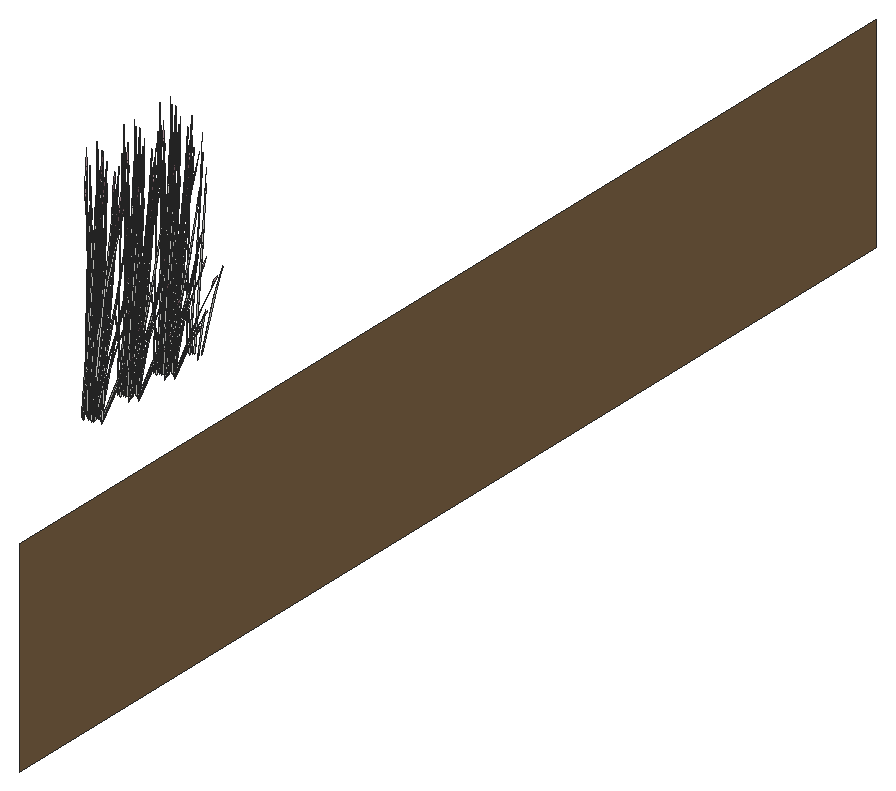
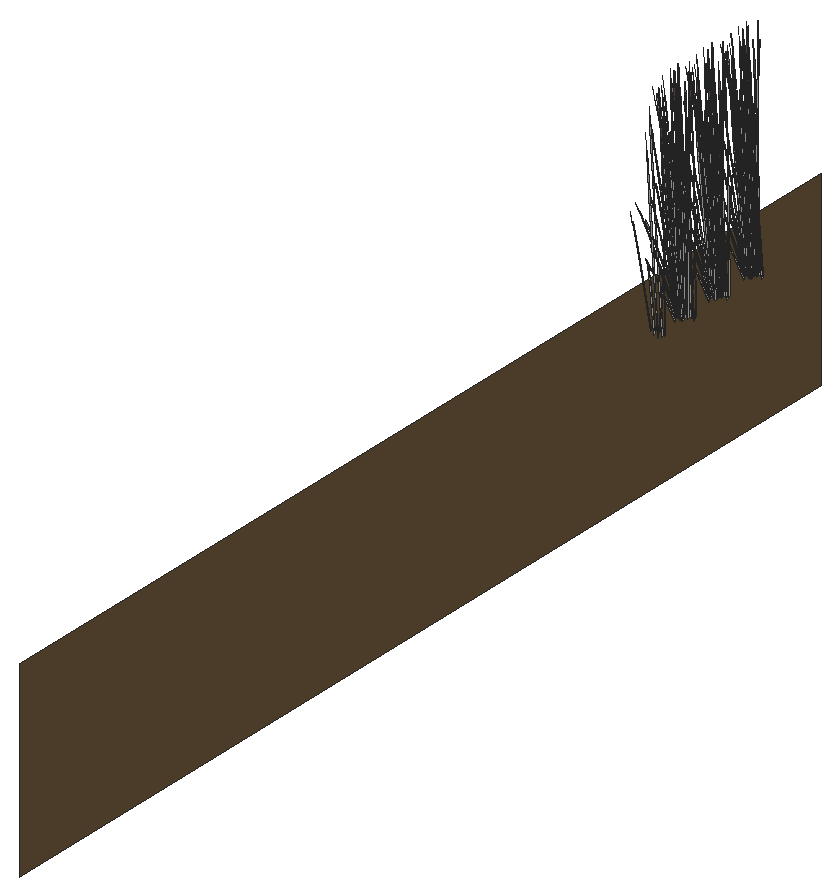
# SketchUp Ruby script. Lengths in inches.
U = 1.inch
M = Sketchup.active_model
def pt(a) = Geom::Point3d.new(a.map { |v| v * U })
def face(e, loops, mat)
  f = e.add_face(loops[0].map { |a| pt(a) })
  loops[1..].each { |l| e.add_face(l.map { |a| pt(a) }).erase! }
  f.material = f.back_material = mat if mat
  f
end
# faces: each face lists its corners as indices into pts; further lists are holes
def faces(e, pts, list, mat = nil) = list.each { |f| face(e, (f[0].is_a?(Array) ? f : [f]).map { |l| l.map { |i| pts[i] } }, mat) }
# xy, xz, yz: faces in a plane at the given z, y or x. An outline is a flat list of corners, or four numbers for a rectangle; further outlines are holes
def ring(l) = l.size == 4 ? [[l[0], l[1]], [l[2], l[1]], [l[2], l[3]], [l[0], l[3]]] : l.each_slice(2).to_a
def flat(e, list, mat, &to3) = list.each { |f| face(e, (f[0].is_a?(Array) ? f : [f]).map { |l| ring(l).map { |u, v| to3.(u, v) } }, mat) }
def xy(e, z, list, mat = nil) = flat(e, list, mat) { |x, y| [x, y, z] }
def xz(e, y, list, mat = nil) = flat(e, list, mat) { |x, z| [x, y, z] }
def yz(e, x, list, mat = nil) = flat(e, list, mat) { |y, z| [x, y, z] }
def lines(e, pts, list) = list.each { |a, b| e.add_line(pt(pts[a]), pt(pts[b])) }
# prism: a flat outline (further loops are holes) pulled along v
def prism(e, loops, v, mat = nil)
  f = face(e, loops, mat); d = Geom::Vector3d.new(v.map { |x| x * U })
  f.pushpull(f.normal.samedirection?(d) ? d.length : -d.length)
end
def box(e, o, s, mat = nil) = prism(e, [[o, [o[0] + s[0], o[1], o[2]], [o[0] + s[0], o[1] + s[1], o[2]], [o[0], o[1] + s[1], o[2]]]], [0, 0, s[2]], mat)
def at(x, y, z, deg = 0) = Geom::Transformation.translation(pt([x, y, z])) * Geom::Transformation.rotation(ORIGIN, Z_AXIS, deg.degrees)
def axes(o, x, y, z) = Geom::Transformation.new([*x, 0, *y, 0, *z, 0, *pt(o).to_a, 1])
def part(name) = M.definitions.add(name)
# library, detail: a bought-in or finely detailed component or shape, given as its bounding box
def library(name, o, s) = part(name).tap { |d| box(d.entities, o, s) }
def detail(e, o, s) = box(e.add_group.entities, o, s)
def put(e, d, t, mat = nil) = e.add_instance(d, t).tap { |i| i.material = mat if mat }
def group(e, t, mat = nil) = e.add_group.tap { |g| g.transformation = t; g.material = mat if mat }.entities
root = M.entities
M.materials.add("LightPink_Translucent").color = [144, 107, 117]
M.materials["LightPink_Translucent"].alpha = 0.75
M.materials.add("Soil_03_1K").color = [122, 96, 67]
c1 = part("blade")
p = [[2.15,0.21,22],[0,0.17,0],[0.09,0.45,0],[2.18,0.31,22],[2.29,0.31,22],[0.38,0.45,0],
  [2.48,0.24,33],[2.49,0.24,33],[2.48,0.22,33]]
faces(c1.entities,p,[[0,1,2,3],[4,5,2,3],[6,3,4,7],[8,0,3,6]])
c2 = part("seeds")
p = [[0.3,-0.1,1.38],[-0.01,-0.03,1.59],[-0.01,-0.03,0.03],[0.14,-0.07,-0.07],[0.29,-0.03,3],[0.15,0.01,3.11]]
faces(c2.entities,p,[[0,1,2,3],[1,0,4,5]],"LightPink_Translucent")
c3 = part("blade with seeds")
put(c3.entities,c1,at(0,0,0))
put(c3.entities,c2,axes([2.4,0.25,30.99],[1.5799,-0.05474,1.17369],[-0.12525,1.92788,0.29478],[-0.07173,-0.02425,1.56792]))
yz(root,352,[[262,0,514,48]],"Soil_03_1K")
put(root,c3,axes([333.35,303.47,49.78],[0.47255,-0.19538,-0.43871],[0.28245,0.35034,0],[0.10763,-0.0445,1.3917]))
put(root,c3,axes([336.15,304.15,50.29],[-0.18038,-0.01157,1.26356],[-0.18479,-0.31048,-0.27174],[0.22159,-0.08783,0.54024]))
put(root,c3,axes([333.91,304.28,49.82],[0.34009,-0.2937,-0.55095],[0.42248,0.26632,-0.1446],[0.13628,-0.07327,1.21613]))
put(root,c3,axes([333.54,304.62,50.36],[-0.05884,-0.44587,-0.25709],[0.6128,-0.02696,-0.44182],[0.10791,-0.05939,1.41118]))
put(root,c3,axes([333.46,303.63,49.79],[0.47106,0.09668,-0.27372],[-0.11861,0.34048,0.27372],[0.09497,-0.03926,1.22797]))
put(root,c3,axes([333.62,304.97,50.15],[0.56891,0.18939,0.21263],[-0.2738,0.39352,0.44182],[0,-0.09071,1.41855]))
put(root,c3,axes([333.44,304.7,50.4],[-0.54829,0.02412,0.39531],[-0.04958,-0.40041,-0.19025],[0.09816,-0.04058,1.26923]))
put(root,c3,axes([335.24,303.63,50.1],[0.31568,-0.39156,0],[0.52815,0.21836,-0.456],[0.12029,0.04973,1.44655]))
put(root,c3,axes([336.49,305.18,49.75],[-0.3252,0.04689,1.25103],[-0.05176,-0.37326,0.07161],[0.22777,-0.0565,0.71188]))
put(root,c3,axes([337.08,304.85,50],[-0.31304,-0.24986,-0.05733],[0.34284,-0.22894,-0.25992],[0.09714,-0.01612,0.85731]))
put(root,c3,axes([334.21,304.88,49.95],[0,-0.45213,0],[0.63136,0,0],[0,0,1.58567]))
put(root,c3,axes([334.97,303.84,50.19],[-0.47255,-0.19538,0.43871],[0.28245,-0.35034,0],[0.10763,0.0445,1.3917]))
put(root,c3,axes([333.91,304.6,50.09],[-0.41865,0.35461,0.40429],[-0.49737,-0.31303,0.15865],[0.10093,-0.03539,1.40366]))
put(root,c3,axes([333.18,304.01,50.1875],[-0.14586,0.38834,0.15589],[-0.53375,-0.1099,0.31002],[0.0922,-0.00189,1.41735]))
put(root,c3,axes([332.96,304.33,49.41],[-0.49699,0.15644,1.13921],[-0.15819,-0.44887,0.44265],[0.30518,0.00747,1.29573]))
put(root,c3,axes([334.29,304.45,50.3125],[0.09741,-0.34873,0.12794],[0.4759,0.06053,-0.36534],[0.08661,0.03581,1.11991]))
put(root,c3,axes([336.84,304.9375,49.32],[-0.02639,-0.05932,1.55816],[0.18302,-0.34702,-0.23804],[0.18462,-0.00499,0.26541]))
put(root,c3,axes([334.09,304.54,50.4],[-0.30332,-0.32798,0.39531],[0.45944,-0.23096,-0.19025],[0.09816,0.04058,1.26923]))
put(root,c3,axes([334.25,304.56,50.36],[0.50979,-0.25942,-0.25709],[0.339,0.36656,-0.44182],[0.12578,0.03723,1.41118]))
put(root,c3,axes([335.53,303.87,49.78],[0.47255,0.19538,-0.43871],[-0.28245,0.35034,0],[0.10763,0.0445,1.3917]))
put(root,c3,axes([334.63,304.98,49.95],[0.56491,0,0],[0,0.40454,0],[0,0,1.5764]))
put(root,c3,axes([334.79,304.04,50.1875],[-0.54257,0.10371,0.15589],[-0.13397,-0.38597,0.31002],[0.04839,0.05624,1.41735]))
put(root,c3,axes([335.4,304.02,49.79],[0.11861,0.34048,-0.27372],[-0.47106,0.09668,0.27372],[0.09497,0.03926,1.22797]))
put(root,c3,axes([334.45,304.78,50.1],[-0.63817,-0.08233,0.43472],[0.12987,-0.46497,0.17059],[0.09326,0.0449,1.50931]))
put(root,c3,axes([334.56,305.88,49.93],[0.53009,-0.13258,-0.16963],[0.18627,0.38191,0.00007],[0.05851,-0.01465,1.53656]))
put(root,c3,axes([334.62,305.16,49.96],[0.35245,0.2524,0],[-0.35245,0.2524,0],[0,0,1.49564]))
put(root,c3,axes([335.58,305.05,50.1875],[-0.39671,-0.28463,0.15589],[0.39978,-0.27607,0.31002],[-0.04381,0.05813,1.41735]))
put(root,c3,axes([334.84,304.62,49.82],[0.52523,0.06406,-0.55095],[-0.11084,0.39517,-0.1446],[0.15674,0.04788,1.21613]))
put(root,c3,axes([334.62,304.86,50.4],[0.24498,-0.3521,0.39531],[0.50902,0.16945,-0.19025],[0,0.08116,1.26923]))
put(root,c3,axes([334.52,305.0625,50.03],[0,0.45191,-0.04981],[-0.63136,0,0],[0,0.0142,1.58489]))
put(root,c3,axes([334.57,304.74,49.95],[0.30332,0.32798,-0.39531],[-0.45944,0.23096,0.19025],[0.09816,0.04058,1.26923]))
put(root,c3,axes([335.9,305.06,50.19],[0,-0.39075,0.43871],[0.56491,0,0],[0,0.089,1.3917]))
put(root,c3,axes([334.83,304.94,50.3125],[0.47043,-0.11396,0.12794],[0.16474,0.32541,-0.36534],[0,0.07162,1.11991]))
put(root,c3,axes([336.58,305.74,50.29],[-0.1216,-0.0961,1.26356],[0.15822,-0.31792,-0.27174],[0.24603,0.04307,0.54024]))
put(root,c3,axes([334.4,306.09,49.95],[0.50902,0.17543,0],[-0.24498,0.36452,0],[0,0,1.54589]))
put(root,c3,axes([334.22,305.9375,50.02],[0.21952,0.44891,-0.05313],[-0.62724,0.1573,0],[0.00767,0.01568,1.52132]))
put(root,c3,axes([336.29,305.125,50.1],[0.63136,0,0],[0,0.43672,-0.456],[0,0.09947,1.44655]))
put(root,c3,axes([336.03,305.35,49.94],[-0.63105,-0.00312,-0.04397],[0,-0.43672,0.44129],[-0.01983,0.09942,1.3992]))
put(root,c3,axes([334.67,304.97,50.36],[0.56863,0.18645,-0.25709],[-0.2738,0.39352,-0.44182],[0.01787,0.09662,1.41118]))
put(root,c3,axes([335.9,305.41,49.79],[-0.35245,0.2438,-0.27372],[-0.35245,-0.2438,0.27372],[0,0.07853,1.22797]))
put(root,c3,axes([336.15,305.42,49.78],[0,0.39075,-0.43871],[-0.56491,0,0],[0,0.089,1.3917]))
put(root,c3,axes([335.51,306.65,49.32],[0.03679,-0.05641,1.55816],[0.46313,-0.16615,-0.23804],[0.14041,0.08599,0.26541]))
put(root,c3,axes([334.9,305.37,49.85],[0.18514,0.35777,-0.61156],[-0.53331,0.12885,-0.16051],[0.02046,0.12115,1.3499]))
put(root,c3,axes([335.47,306.74,50.36],[-0.32378,-0.01225,0.92831],[0.21383,-0.26028,0.51254],[0.12791,0.09247,0.72818]))
put(root,c3,axes([334.42,306.11,50.29],[0.00891,-0.12953,1.26356],[0.4258,-0.14469,-0.27174],[0.13144,0.15503,0.54024]))
put(root,c3,axes([334.77,314.21,50.29],[-0.14352,0.07909,1.26356],[-0.42983,-0.13843,-0.27174],[0.07968,-0.17216,0.54024]))
put(root,c3,axes([335.77,314.45,49.32],[-0.07557,-0.03078,1.55816],[-0.19412,-0.34391,-0.23804],[0.13095,-0.09333,0.26541]))
put(root,c3,axes([332.92,314.52,50.1],[-0.31568,-0.39156,0],[0.52815,-0.21836,-0.456],[0.12029,-0.04973,1.44655]))
put(root,c3,axes([333.35,314.46,49.78],[0.47255,-0.19538,-0.43871],[0.28245,0.35034,0],[0.10763,-0.0445,1.3917]))
put(root,c3,axes([336.15,315.14,50.29],[-0.18038,-0.01157,1.26356],[-0.18479,-0.31048,-0.27174],[0.22159,-0.08783,0.54024]))
put(root,c3,axes([333.91,315.26,49.82],[0.34009,-0.2937,-0.55095],[0.42248,0.26632,-0.1446],[0.13628,-0.07327,1.21613]))
put(root,c3,axes([333.54,315.61,50.36],[-0.05884,-0.44587,-0.25709],[0.6128,-0.02696,-0.44182],[0.10791,-0.05939,1.41118]))
put(root,c3,axes([333.46,314.62,49.79],[0.47106,0.09668,-0.27372],[-0.11861,0.34048,0.27372],[0.09497,-0.03926,1.22797]))
put(root,c3,axes([333.62,315.95,50.15],[0.56891,0.18939,0.21263],[-0.2738,0.39352,0.44182],[0,-0.09071,1.41855]))
put(root,c3,axes([333.44,315.69,50.4],[-0.54829,0.02412,0.39531],[-0.04958,-0.40041,-0.19025],[0.09816,-0.04058,1.26923]))
put(root,c3,axes([335.24,314.62,50.1],[0.31568,-0.39156,0],[0.52815,0.21836,-0.456],[0.12029,0.04973,1.44655]))
put(root,c3,axes([336.49,316.17,49.75],[-0.3252,0.04689,1.25103],[-0.05176,-0.37326,0.07161],[0.22777,-0.0565,0.71188]))
put(root,c3,axes([337.08,315.84,50],[-0.31304,-0.24986,-0.05733],[0.34284,-0.22894,-0.25992],[0.09714,-0.01612,0.85731]))
put(root,c3,axes([334.21,315.87,49.95],[0,-0.45213,0],[0.63136,0,0],[0,0,1.58567]))
put(root,c3,axes([334.97,314.83,50.19],[-0.47255,-0.19538,0.43871],[0.28245,-0.35034,0],[0.10763,0.0445,1.3917]))
put(root,c3,axes([333.91,315.59,50.09],[-0.41865,0.35461,0.40429],[-0.49737,-0.31303,0.15865],[0.10093,-0.03539,1.40366]))
put(root,c3,axes([333.18,315,50.1875],[-0.14586,0.38834,0.15589],[-0.53375,-0.1099,0.31002],[0.0922,-0.00189,1.41735]))
put(root,c3,axes([332.96,315.32,49.41],[-0.49699,0.15644,1.13921],[-0.15819,-0.44887,0.44265],[0.30518,0.00747,1.29573]))
put(root,c3,axes([334.29,315.43,50.3125],[0.09741,-0.34873,0.12794],[0.4759,0.06053,-0.36534],[0.08661,0.03581,1.11991]))
put(root,c3,axes([336.84,315.93,49.32],[-0.02639,-0.05932,1.55816],[0.18302,-0.34702,-0.23804],[0.18462,-0.00499,0.26541]))
put(root,c3,axes([334.09,315.53,50.4],[-0.30332,-0.32798,0.39531],[0.45944,-0.23096,-0.19025],[0.09816,0.04058,1.26923]))
put(root,c3,axes([334.25,315.55,50.36],[0.50979,-0.25942,-0.25709],[0.339,0.36656,-0.44182],[0.12578,0.03723,1.41118]))
put(root,c3,axes([335.53,314.86,49.78],[0.47255,0.19538,-0.43871],[-0.28245,0.35034,0],[0.10763,0.0445,1.3917]))
put(root,c3,axes([334.63,315.97,49.95],[0.56491,0,0],[0,0.40454,0],[0,0,1.5764]))
put(root,c3,axes([334.79,315.02,50.1875],[-0.54257,0.10371,0.15589],[-0.13397,-0.38597,0.31002],[0.04839,0.05624,1.41735]))
put(root,c3,axes([335.4,315,49.79],[0.11861,0.34048,-0.27372],[-0.47106,0.09668,0.27372],[0.09497,0.03926,1.22797]))
put(root,c3,axes([334.45,315.77,50.1],[-0.63817,-0.08233,0.43472],[0.12987,-0.46497,0.17059],[0.09326,0.0449,1.50931]))
put(root,c3,axes([334.56,316.87,49.93],[0.53009,-0.13258,-0.16963],[0.18627,0.38191,0.00007],[0.05851,-0.01465,1.53656]))
put(root,c3,axes([334.62,316.15,49.96],[0.35245,0.2524,0],[-0.35245,0.2524,0],[0,0,1.49564]))
put(root,c3,axes([335.58,316.04,50.1875],[-0.39671,-0.28463,0.15589],[0.39978,-0.27607,0.31002],[-0.04381,0.05813,1.41735]))
put(root,c3,axes([334.84,315.61,49.82],[0.52523,0.06406,-0.55095],[-0.11084,0.39517,-0.1446],[0.15674,0.04788,1.21613]))
put(root,c3,axes([334.62,315.85,50.4],[0.24498,-0.3521,0.39531],[0.50902,0.16945,-0.19025],[0,0.08116,1.26923]))
put(root,c3,axes([334.52,316.05,50.03],[0,0.45191,-0.04981],[-0.63136,0,0],[0,0.0142,1.58489]))
put(root,c3,axes([334.57,315.73,49.95],[0.30332,0.32798,-0.39531],[-0.45944,0.23096,0.19025],[0.09816,0.04058,1.26923]))
put(root,c3,axes([335.9,316.05,50.19],[0,-0.39075,0.43871],[0.56491,0,0],[0,0.089,1.3917]))
put(root,c3,axes([334.83,315.93,50.3125],[0.47043,-0.11396,0.12794],[0.16474,0.32541,-0.36534],[0,0.07162,1.11991]))
put(root,c3,axes([336.58,316.72,50.29],[-0.1216,-0.0961,1.26356],[0.15822,-0.31792,-0.27174],[0.24603,0.04307,0.54024]))
put(root,c3,axes([334.4,317.07,49.95],[0.50902,0.17543,0],[-0.24498,0.36452,0],[0,0,1.54589]))
put(root,c3,axes([334.22,316.93,50.02],[0.21952,0.44891,-0.05313],[-0.62724,0.1573,0],[0.00767,0.01568,1.52132]))
put(root,c3,axes([336.29,316.11,50.1],[0.63136,0,0],[0,0.43672,-0.456],[0,0.09947,1.44655]))
put(root,c3,axes([336.03,316.34,49.94],[-0.63105,-0.00312,-0.04397],[0,-0.43672,0.44129],[-0.01983,0.09942,1.3992]))
put(root,c3,axes([334.67,315.96,50.36],[0.56863,0.18645,-0.25709],[-0.2738,0.39352,-0.44182],[0.01787,0.09662,1.41118]))
put(root,c3,axes([335.9,316.4,49.79],[-0.35245,0.2438,-0.27372],[-0.35245,-0.2438,0.27372],[0,0.07853,1.22797]))
put(root,c3,axes([336.15,316.41,49.78],[0,0.39075,-0.43871],[-0.56491,0,0],[0,0.089,1.3917]))
put(root,c3,axes([335.51,317.64,49.32],[0.03679,-0.05641,1.55816],[0.46313,-0.16615,-0.23804],[0.14041,0.08599,0.26541]))
put(root,c3,axes([334.9,316.36,49.85],[0.18514,0.35777,-0.61156],[-0.53331,0.12885,-0.16051],[0.02046,0.12115,1.3499]))
put(root,c3,axes([335.47,317.73,50.36],[-0.32378,-0.01225,0.92831],[0.21383,-0.26028,0.51254],[0.12791,0.09247,0.72818]))
put(root,c3,axes([334.42,317.1,50.29],[0.00891,-0.12953,1.26356],[0.4258,-0.14469,-0.27174],[0.13144,0.15503,0.54024]))
put(root,c3,axes([334.77,324.81,50.29],[-0.14352,0.07909,1.26356],[-0.42983,-0.13843,-0.27174],[0.07968,-0.17216,0.54024]))
put(root,c3,axes([335.77,325.05,49.32],[-0.07557,-0.03078,1.55816],[-0.19412,-0.34391,-0.23804],[0.13095,-0.09333,0.26541]))
put(root,c3,axes([332.92,325.12,50.1],[-0.31568,-0.39156,0],[0.52815,-0.21836,-0.456],[0.12029,-0.04973,1.44655]))
put(root,c3,axes([333.35,325.0625,49.78],[0.47255,-0.19538,-0.43871],[0.28245,0.35034,0],[0.10763,-0.0445,1.3917]))
put(root,c3,axes([336.15,325.74,50.29],[-0.18038,-0.01157,1.26356],[-0.18479,-0.31048,-0.27174],[0.22159,-0.08783,0.54024]))
put(root,c3,axes([333.91,325.86,49.82],[0.34009,-0.2937,-0.55095],[0.42248,0.26632,-0.1446],[0.13628,-0.07327,1.21613]))
put(root,c3,axes([333.54,326.2,50.36],[-0.05884,-0.44587,-0.25709],[0.6128,-0.02696,-0.44182],[0.10791,-0.05939,1.41118]))
put(root,c3,axes([333.46,325.22,49.79],[0.47106,0.09668,-0.27372],[-0.11861,0.34048,0.27372],[0.09497,-0.03926,1.22797]))
put(root,c3,axes([333.62,326.55,50.15],[0.56891,0.18939,0.21263],[-0.2738,0.39352,0.44182],[0,-0.09071,1.41855]))
put(root,c3,axes([333.44,326.29,50.4],[-0.54829,0.02412,0.39531],[-0.04958,-0.40041,-0.19025],[0.09816,-0.04058,1.26923]))
put(root,c3,axes([335.24,325.22,50.1],[0.31568,-0.39156,0],[0.52815,0.21836,-0.456],[0.12029,0.04973,1.44655]))
put(root,c3,axes([336.49,326.77,49.75],[-0.3252,0.04689,1.25103],[-0.05176,-0.37326,0.07161],[0.22777,-0.0565,0.71188]))
put(root,c3,axes([337.08,326.4375,50],[-0.31304,-0.24986,-0.05733],[0.34284,-0.22894,-0.25992],[0.09714,-0.01612,0.85731]))
put(root,c3,axes([334.21,326.47,49.95],[0,-0.45213,0],[0.63136,0,0],[0,0,1.58567]))
put(root,c3,axes([334.97,325.42,50.19],[-0.47255,-0.19538,0.43871],[0.28245,-0.35034,0],[0.10763,0.0445,1.3917]))
put(root,c3,axes([333.91,326.18,50.09],[-0.41865,0.35461,0.40429],[-0.49737,-0.31303,0.15865],[0.10093,-0.03539,1.40366]))
put(root,c3,axes([333.18,325.6,50.1875],[-0.14586,0.38834,0.15589],[-0.53375,-0.1099,0.31002],[0.0922,-0.00189,1.41735]))
put(root,c3,axes([332.96,325.91,49.41],[-0.49699,0.15644,1.13921],[-0.15819,-0.44887,0.44265],[0.30518,0.00747,1.29573]))
put(root,c3,axes([334.29,326.03,50.3125],[0.09741,-0.34873,0.12794],[0.4759,0.06053,-0.36534],[0.08661,0.03581,1.11991]))
put(root,c3,axes([336.84,326.52,49.32],[-0.02639,-0.05932,1.55816],[0.18302,-0.34702,-0.23804],[0.18462,-0.00499,0.26541]))
put(root,c3,axes([334.09,326.125,50.4],[-0.30332,-0.32798,0.39531],[0.45944,-0.23096,-0.19025],[0.09816,0.04058,1.26923]))
put(root,c3,axes([334.25,326.15,50.36],[0.50979,-0.25942,-0.25709],[0.339,0.36656,-0.44182],[0.12578,0.03723,1.41118]))
put(root,c3,axes([335.53,325.46,49.78],[0.47255,0.19538,-0.43871],[-0.28245,0.35034,0],[0.10763,0.0445,1.3917]))
put(root,c3,axes([334.63,326.57,49.95],[0.56491,0,0],[0,0.40454,0],[0,0,1.5764]))
put(root,c3,axes([334.79,325.62,50.1875],[-0.54257,0.10371,0.15589],[-0.13397,-0.38597,0.31002],[0.04839,0.05624,1.41735]))
put(root,c3,axes([335.4,325.6,49.79],[0.11861,0.34048,-0.27372],[-0.47106,0.09668,0.27372],[0.09497,0.03926,1.22797]))
put(root,c3,axes([334.45,326.36,50.1],[-0.63817,-0.08233,0.43472],[0.12987,-0.46497,0.17059],[0.09326,0.0449,1.50931]))
put(root,c3,axes([334.56,327.47,49.93],[0.53009,-0.13258,-0.16963],[0.18627,0.38191,0.00007],[0.05851,-0.01465,1.53656]))
put(root,c3,axes([334.62,326.74,49.96],[0.35245,0.2524,0],[-0.35245,0.2524,0],[0,0,1.49564]))
put(root,c3,axes([335.58,326.63,50.1875],[-0.39671,-0.28463,0.15589],[0.39978,-0.27607,0.31002],[-0.04381,0.05813,1.41735]))
put(root,c3,axes([334.84,326.2,49.82],[0.52523,0.06406,-0.55095],[-0.11084,0.39517,-0.1446],[0.15674,0.04788,1.21613]))
put(root,c3,axes([334.62,326.45,50.4],[0.24498,-0.3521,0.39531],[0.50902,0.16945,-0.19025],[0,0.08116,1.26923]))
put(root,c3,axes([334.52,326.65,50.03],[0,0.45191,-0.04981],[-0.63136,0,0],[0,0.0142,1.58489]))
put(root,c3,axes([334.57,326.33,49.95],[0.30332,0.32798,-0.39531],[-0.45944,0.23096,0.19025],[0.09816,0.04058,1.26923]))
put(root,c3,axes([335.9,326.65,50.19],[0,-0.39075,0.43871],[0.56491,0,0],[0,0.089,1.3917]))
put(root,c3,axes([334.83,326.53,50.3125],[0.47043,-0.11396,0.12794],[0.16474,0.32541,-0.36534],[0,0.07162,1.11991]))
put(root,c3,axes([336.58,327.32,50.29],[-0.1216,-0.0961,1.26356],[0.15822,-0.31792,-0.27174],[0.24603,0.04307,0.54024]))
put(root,c3,axes([334.4,327.67,49.95],[0.50902,0.17543,0],[-0.24498,0.36452,0],[0,0,1.54589]))
put(root,c3,axes([334.22,327.52,50.02],[0.21952,0.44891,-0.05313],[-0.62724,0.1573,0],[0.00767,0.01568,1.52132]))
put(root,c3,axes([336.29,326.71,50.1],[0.63136,0,0],[0,0.43672,-0.456],[0,0.09947,1.44655]))
put(root,c3,axes([336.03,326.9375,49.94],[-0.63105,-0.00312,-0.04397],[0,-0.43672,0.44129],[-0.01983,0.09942,1.3992]))
put(root,c3,axes([334.67,326.56,50.36],[0.56863,0.18645,-0.25709],[-0.2738,0.39352,-0.44182],[0.01787,0.09662,1.41118]))
put(root,c3,axes([335.9,327,49.79],[-0.35245,0.2438,-0.27372],[-0.35245,-0.2438,0.27372],[0,0.07853,1.22797]))
put(root,c3,axes([336.15,327.01,49.78],[0,0.39075,-0.43871],[-0.56491,0,0],[0,0.089,1.3917]))
put(root,c3,axes([335.51,328.24,49.32],[0.03679,-0.05641,1.55816],[0.46313,-0.16615,-0.23804],[0.14041,0.08599,0.26541]))
put(root,c3,axes([334.9,326.95,49.85],[0.18514,0.35777,-0.61156],[-0.53331,0.12885,-0.16051],[0.02046,0.12115,1.3499]))
put(root,c3,axes([335.47,328.33,50.36],[-0.32378,-0.01225,0.92831],[0.21383,-0.26028,0.51254],[0.12791,0.09247,0.72818]))
put(root,c3,axes([334.42,327.7,50.29],[0.00891,-0.12953,1.26356],[0.4258,-0.14469,-0.27174],[0.13144,0.15503,0.54024]))
put(root,c3,axes([334.77,334.51,50.29],[-0.14352,0.07909,1.26356],[-0.42983,-0.13843,-0.27174],[0.07968,-0.17216,0.54024]))
put(root,c3,axes([335.77,334.75,49.32],[-0.07557,-0.03078,1.55816],[-0.19412,-0.34391,-0.23804],[0.13095,-0.09333,0.26541]))
put(root,c3,axes([332.92,334.83,50.1],[-0.31568,-0.39156,0],[0.52815,-0.21836,-0.456],[0.12029,-0.04973,1.44655]))
put(root,c3,axes([333.35,334.77,49.78],[0.47255,-0.19538,-0.43871],[0.28245,0.35034,0],[0.10763,-0.0445,1.3917]))
put(root,c3,axes([336.15,335.44,50.29],[-0.18038,-0.01157,1.26356],[-0.18479,-0.31048,-0.27174],[0.22159,-0.08783,0.54024]))
put(root,c3,axes([333.91,335.57,49.82],[0.34009,-0.2937,-0.55095],[0.42248,0.26632,-0.1446],[0.13628,-0.07327,1.21613]))
